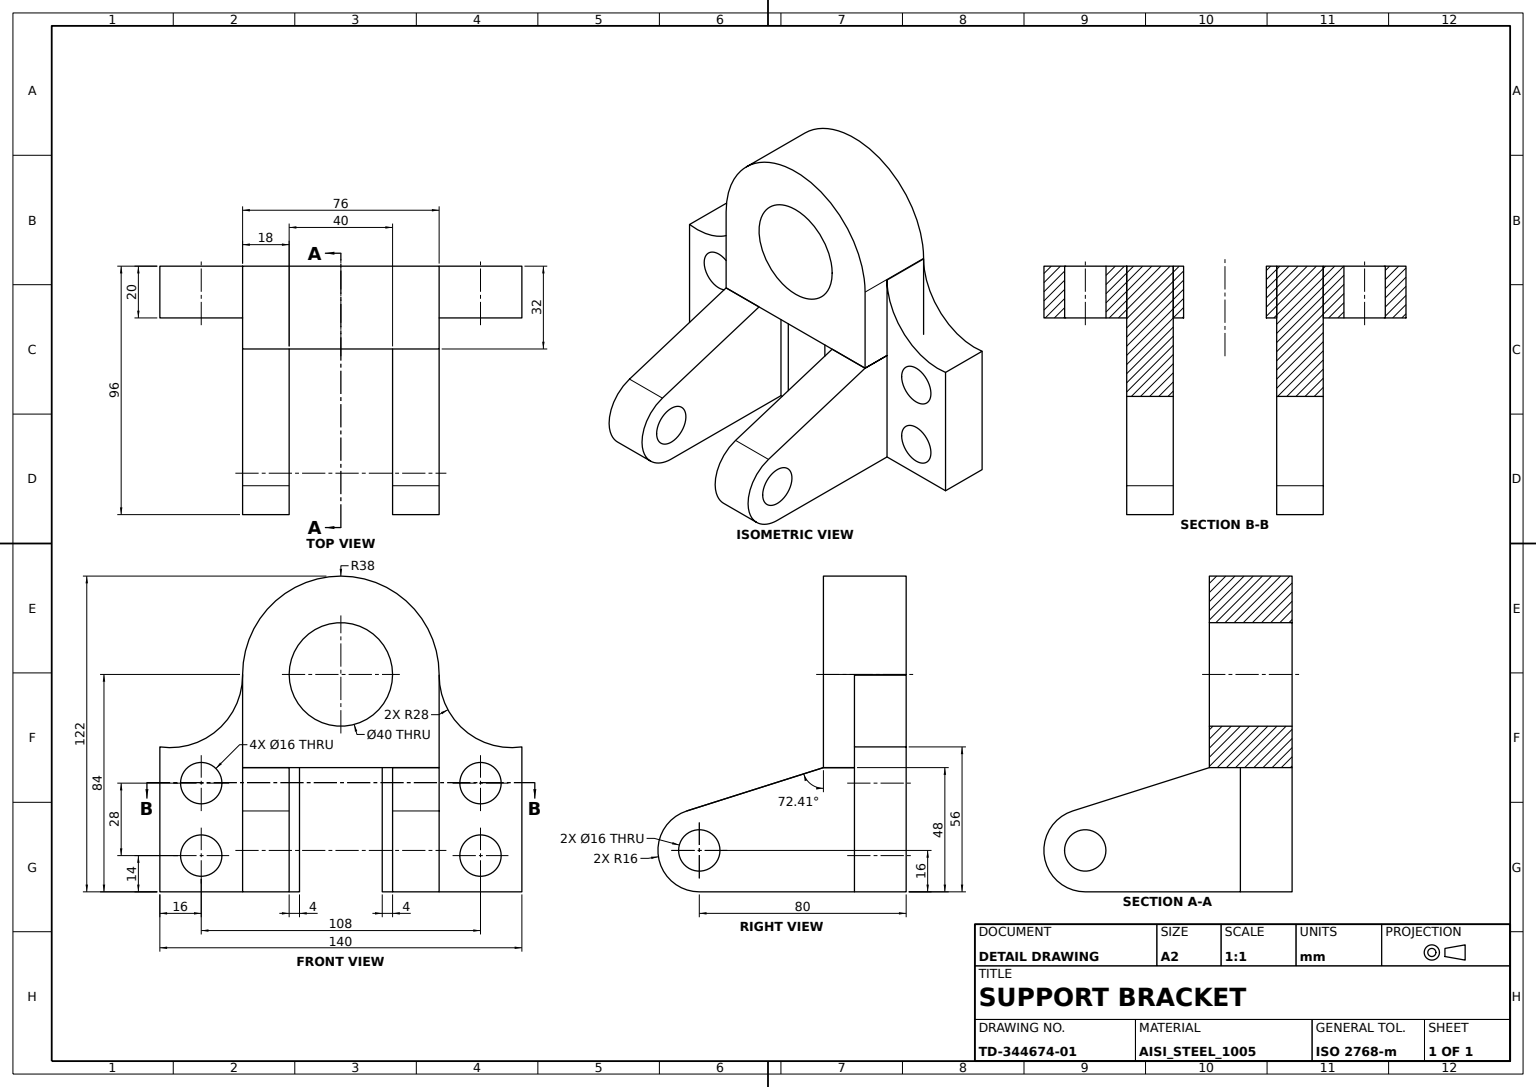
ISO-10303-21;
HEADER;
FILE_DESCRIPTION((''),'2;1');
FILE_NAME('','',(''),(''),'','','');
FILE_SCHEMA(('AUTOMOTIVE_DESIGN'));
ENDSEC;
DATA;
#1=APPLICATION_CONTEXT('');
#2=PRODUCT_CONTEXT('',#1,'mechanical');
#3=PRODUCT('','','',(#2));
#4=PRODUCT_DEFINITION_FORMATION('','',#3);
#5=PRODUCT_DEFINITION_CONTEXT('',#1,'design');
#6=PRODUCT_DEFINITION('','',#4,#5);
#7=PRODUCT_DEFINITION_SHAPE('','',#6);
#8=(LENGTH_UNIT()NAMED_UNIT(*)SI_UNIT(.MILLI.,.METRE.));
#9=(NAMED_UNIT(*)PLANE_ANGLE_UNIT()SI_UNIT($,.RADIAN.));
#10=(NAMED_UNIT(*)SI_UNIT($,.STERADIAN.)SOLID_ANGLE_UNIT());
#11=UNCERTAINTY_MEASURE_WITH_UNIT(LENGTH_MEASURE(0.005),#8,'distance_accuracy_value','');
#12=(GEOMETRIC_REPRESENTATION_CONTEXT(3)GLOBAL_UNCERTAINTY_ASSIGNED_CONTEXT((#11))GLOBAL_UNIT_ASSIGNED_CONTEXT((#8,#9,#10))REPRESENTATION_CONTEXT('',''));
#13=CARTESIAN_POINT('',(20.,-38.,-84.));
#14=VERTEX_POINT('',#13);
#15=CARTESIAN_POINT('',(20.,-70.,-84.));
#16=VERTEX_POINT('',#15);
#17=DIRECTION('',(0.,-1.,0.));
#18=VECTOR('',#17,1000.);
#19=LINE('',#13,#18);
#20=EDGE_CURVE('',#14,#16,#19,.T.);
#21=ORIENTED_EDGE('',*,*,#20,.T.);
#22=CARTESIAN_POINT('',(0.,-70.,-84.));
#23=VERTEX_POINT('',#22);
#24=DIRECTION('',(-1.,0.,0.));
#25=VECTOR('',#24,1000.);
#26=LINE('',#15,#25);
#27=EDGE_CURVE('',#16,#23,#26,.T.);
#28=ORIENTED_EDGE('',*,*,#27,.T.);
#29=CARTESIAN_POINT('',(0.,-38.,-84.));
#30=VERTEX_POINT('',#29);
#31=LINE('',#29,#18);
#32=EDGE_CURVE('',#30,#23,#31,.T.);
#33=ORIENTED_EDGE('',*,*,#32,.F.);
#34=LINE('',#13,#25);
#35=EDGE_CURVE('',#14,#30,#34,.T.);
#36=ORIENTED_EDGE('',*,*,#35,.F.);
#37=EDGE_LOOP('',(#21,#28,#33,#36));
#38=FACE_BOUND('',#37,.T.);
#39=DIRECTION('',(0.,0.,-1.));
#40=AXIS2_PLACEMENT_3D('',#13,#39,#24);
#41=PLANE('',#40);
#42=ADVANCED_FACE('',(#38),#41,.T.);
#43=CARTESIAN_POINT('',(20.,-70.,-28.));
#44=VERTEX_POINT('',#43);
#45=CARTESIAN_POINT('',(0.,-70.,-28.));
#46=VERTEX_POINT('',#45);
#47=LINE('',#43,#25);
#48=EDGE_CURVE('',#44,#46,#47,.T.);
#49=ORIENTED_EDGE('',*,*,#48,.T.);
#50=DIRECTION('',(0.,0.,1.));
#51=VECTOR('',#50,1000.);
#52=LINE('',#22,#51);
#53=EDGE_CURVE('',#23,#46,#52,.T.);
#54=ORIENTED_EDGE('',*,*,#53,.F.);
#55=ORIENTED_EDGE('',*,*,#27,.F.);
#56=LINE('',#15,#51);
#57=EDGE_CURVE('',#16,#44,#56,.T.);
#58=ORIENTED_EDGE('',*,*,#57,.T.);
#59=EDGE_LOOP('',(#49,#54,#55,#58));
#60=FACE_BOUND('',#59,.T.);
#61=AXIS2_PLACEMENT_3D('',#15,#17,#39);
#62=PLANE('',#61);
#63=ADVANCED_FACE('',(#60),#62,.T.);
#64=CARTESIAN_POINT('',(20.,-38.,-0.287187));
#65=VERTEX_POINT('',#64);
#66=CARTESIAN_POINT('',(0.,-38.,-0.287187));
#67=VERTEX_POINT('',#66);
#68=LINE('',#64,#25);
#69=EDGE_CURVE('',#65,#67,#68,.T.);
#70=ORIENTED_EDGE('',*,*,#69,.T.);
#71=CARTESIAN_POINT('',(0.,-66.,-0.287187));
#72=DIRECTION('',(1.,0.,0.));
#73=AXIS2_PLACEMENT_3D('',#71,#72,#17);
#74=CIRCLE('',#73,28.);
#75=EDGE_CURVE('',#46,#67,#74,.T.);
#76=ORIENTED_EDGE('',*,*,#75,.F.);
#77=ORIENTED_EDGE('',*,*,#48,.F.);
#78=CARTESIAN_POINT('',(20.,-66.,-0.287187));
#79=AXIS2_PLACEMENT_3D('',#78,#72,#17);
#80=CIRCLE('',#79,28.);
#81=EDGE_CURVE('',#44,#65,#80,.T.);
#82=ORIENTED_EDGE('',*,*,#81,.T.);
#83=EDGE_LOOP('',(#70,#76,#77,#82));
#84=FACE_BOUND('',#83,.T.);
#85=AXIS2_PLACEMENT_3D('',#78,#24,#50);
#86=CYLINDRICAL_SURFACE('',#85,28.);
#87=ADVANCED_FACE('',(#84),#86,.F.);
#88=ORIENTED_EDGE('',*,*,#69,.F.);
#89=VECTOR('',#39,1000.);
#90=LINE('',#64,#89);
#91=EDGE_CURVE('',#65,#14,#90,.T.);
#92=ORIENTED_EDGE('',*,*,#91,.T.);
#93=ORIENTED_EDGE('',*,*,#35,.T.);
#94=CARTESIAN_POINT('',(0.,-38.,-36.));
#95=LINE('',#94,#89);
#96=EDGE_CURVE('',#67,#30,#95,.T.);
#97=ORIENTED_EDGE('',*,*,#96,.F.);
#98=EDGE_LOOP('',(#88,#92,#93,#97));
#99=FACE_BOUND('',#98,.T.);
#100=CARTESIAN_POINT('',(20.,-38.,-36.));
#101=DIRECTION('',(0.,1.,0.));
#102=AXIS2_PLACEMENT_3D('',#100,#101,#50);
#103=PLANE('',#102);
#104=ADVANCED_FACE('',(#99),#103,.T.);
#105=CARTESIAN_POINT('',(0.,-46.,-42.));
#106=VERTEX_POINT('',#105);
#107=CARTESIAN_POINT('',(0.,-54.,-42.));
#108=AXIS2_PLACEMENT_3D('',#107,#24,#101);
#109=CIRCLE('',#108,8.);
#110=EDGE_CURVE('',#106,#106,#109,.T.);
#111=ORIENTED_EDGE('',*,*,#110,.T.);
#112=EDGE_LOOP('',(#111));
#113=FACE_BOUND('',#112,.T.);
#114=CARTESIAN_POINT('',(20.,-46.,-42.));
#115=VERTEX_POINT('',#114);
#116=CARTESIAN_POINT('',(20.,-54.,-42.));
#117=AXIS2_PLACEMENT_3D('',#116,#24,#101);
#118=CIRCLE('',#117,8.);
#119=EDGE_CURVE('',#115,#115,#118,.T.);
#120=ORIENTED_EDGE('',*,*,#119,.F.);
#121=EDGE_LOOP('',(#120));
#122=FACE_BOUND('',#121,.T.);
#123=AXIS2_PLACEMENT_3D('',#107,#72,#39);
#124=CYLINDRICAL_SURFACE('',#123,8.);
#125=ADVANCED_FACE('',(#113,#122),#124,.F.);
#126=CARTESIAN_POINT('',(20.,-46.,-70.));
#127=VERTEX_POINT('',#126);
#128=CARTESIAN_POINT('',(20.,-54.,-70.));
#129=AXIS2_PLACEMENT_3D('',#128,#24,#101);
#130=CIRCLE('',#129,8.);
#131=EDGE_CURVE('',#127,#127,#130,.T.);
#132=ORIENTED_EDGE('',*,*,#131,.T.);
#133=EDGE_LOOP('',(#132));
#134=FACE_BOUND('',#133,.T.);
#135=ORIENTED_EDGE('',*,*,#119,.T.);
#136=EDGE_LOOP('',(#135));
#137=FACE_BOUND('',#136,.T.);
#138=ORIENTED_EDGE('',*,*,#57,.F.);
#139=ORIENTED_EDGE('',*,*,#20,.F.);
#140=ORIENTED_EDGE('',*,*,#91,.F.);
#141=ORIENTED_EDGE('',*,*,#81,.F.);
#142=EDGE_LOOP('',(#138,#139,#140,#141));
#143=FACE_BOUND('',#142,.T.);
#144=AXIS2_PLACEMENT_3D('',#78,#72,#39);
#145=PLANE('',#144);
#146=ADVANCED_FACE('',(#134,#137,#143),#145,.T.);
#147=ORIENTED_EDGE('',*,*,#131,.F.);
#148=EDGE_LOOP('',(#147));
#149=FACE_BOUND('',#148,.T.);
#150=CARTESIAN_POINT('',(0.,-46.,-70.));
#151=VERTEX_POINT('',#150);
#152=CARTESIAN_POINT('',(0.,-54.,-70.));
#153=AXIS2_PLACEMENT_3D('',#152,#24,#101);
#154=CIRCLE('',#153,8.);
#155=EDGE_CURVE('',#151,#151,#154,.T.);
#156=ORIENTED_EDGE('',*,*,#155,.T.);
#157=EDGE_LOOP('',(#156));
#158=FACE_BOUND('',#157,.T.);
#159=AXIS2_PLACEMENT_3D('',#152,#72,#39);
#160=CYLINDRICAL_SURFACE('',#159,8.);
#161=ADVANCED_FACE('',(#149,#158),#160,.F.);
#162=ORIENTED_EDGE('',*,*,#75,.T.);
#163=ORIENTED_EDGE('',*,*,#96,.T.);
#164=ORIENTED_EDGE('',*,*,#32,.T.);
#165=ORIENTED_EDGE('',*,*,#53,.T.);
#166=EDGE_LOOP('',(#162,#163,#164,#165));
#167=FACE_BOUND('',#166,.T.);
#168=ORIENTED_EDGE('',*,*,#155,.F.);
#169=EDGE_LOOP('',(#168));
#170=FACE_BOUND('',#169,.T.);
#171=ORIENTED_EDGE('',*,*,#110,.F.);
#172=EDGE_LOOP('',(#171));
#173=FACE_BOUND('',#172,.T.);
#174=AXIS2_PLACEMENT_3D('',#71,#72,#39);
#175=PLANE('',#174);
#176=ADVANCED_FACE('',(#167,#170,#173),#175,.F.);
#177=CLOSED_SHELL('',(#42,#63,#87,#104,#125,#146,#161,#176));
#178=MANIFOLD_SOLID_BREP('',#177);
#179=CARTESIAN_POINT('',(0.,-20.,-84.));
#180=VERTEX_POINT('',#179);
#181=CARTESIAN_POINT('',(0.,-20.,-36.));
#182=VERTEX_POINT('',#181);
#183=LINE('',#179,#51);
#184=EDGE_CURVE('',#180,#182,#183,.T.);
#185=ORIENTED_EDGE('',*,*,#184,.F.);
#186=VERTEX_POINT('',#29);
#187=LINE('',#179,#18);
#188=EDGE_CURVE('',#180,#186,#187,.T.);
#189=ORIENTED_EDGE('',*,*,#188,.T.);
#190=VERTEX_POINT('',#94);
#191=LINE('',#29,#51);
#192=EDGE_CURVE('',#186,#190,#191,.T.);
#193=ORIENTED_EDGE('',*,*,#192,.T.);
#194=LINE('',#181,#18);
#195=EDGE_CURVE('',#182,#190,#194,.T.);
#196=ORIENTED_EDGE('',*,*,#195,.F.);
#197=EDGE_LOOP('',(#185,#189,#193,#196));
#198=FACE_BOUND('',#197,.T.);
#199=AXIS2_PLACEMENT_3D('',#179,#72,#39);
#200=PLANE('',#199);
#201=ADVANCED_FACE('',(#198),#200,.F.);
#202=CARTESIAN_POINT('',(84.834712,-20.,-52.747932));
#203=VERTEX_POINT('',#202);
#204=CARTESIAN_POINT('',(84.834712,-38.,-52.747932));
#205=VERTEX_POINT('',#204);
#206=LINE('',#202,#18);
#207=EDGE_CURVE('',#203,#205,#206,.T.);
#208=ORIENTED_EDGE('',*,*,#207,.T.);
#209=CARTESIAN_POINT('',(80.,-38.,-84.));
#210=VERTEX_POINT('',#209);
#211=CARTESIAN_POINT('',(80.,-38.,-68.));
#212=AXIS2_PLACEMENT_3D('',#211,#101,#72);
#213=CIRCLE('',#212,16.);
#214=EDGE_CURVE('',#205,#210,#213,.T.);
#215=ORIENTED_EDGE('',*,*,#214,.T.);
#216=CARTESIAN_POINT('',(80.,-20.,-84.));
#217=VERTEX_POINT('',#216);
#218=LINE('',#216,#18);
#219=EDGE_CURVE('',#217,#210,#218,.T.);
#220=ORIENTED_EDGE('',*,*,#219,.F.);
#221=CARTESIAN_POINT('',(80.,-20.,-68.));
#222=AXIS2_PLACEMENT_3D('',#221,#101,#72);
#223=CIRCLE('',#222,16.);
#224=EDGE_CURVE('',#203,#217,#223,.T.);
#225=ORIENTED_EDGE('',*,*,#224,.F.);
#226=EDGE_LOOP('',(#208,#215,#220,#225));
#227=FACE_BOUND('',#226,.T.);
#228=AXIS2_PLACEMENT_3D('',#221,#17,#39);
#229=CYLINDRICAL_SURFACE('',#228,16.);
#230=ADVANCED_FACE('',(#227),#229,.T.);
#231=CARTESIAN_POINT('',(88.,-20.,-68.));
#232=VERTEX_POINT('',#231);
#233=CIRCLE('',#222,8.);
#234=EDGE_CURVE('',#232,#232,#233,.T.);
#235=ORIENTED_EDGE('',*,*,#234,.F.);
#236=EDGE_LOOP('',(#235));
#237=FACE_BOUND('',#236,.T.);
#238=ORIENTED_EDGE('',*,*,#184,.T.);
#239=CARTESIAN_POINT('',(32.,-20.,-36.));
#240=VERTEX_POINT('',#239);
#241=VECTOR('',#72,1000.);
#242=LINE('',#181,#241);
#243=EDGE_CURVE('',#182,#240,#242,.T.);
#244=ORIENTED_EDGE('',*,*,#243,.T.);
#245=DIRECTION('',(0.953254219,0.,-0.302169479));
#246=VECTOR('',#245,1000.);
#247=LINE('',#239,#246);
#248=EDGE_CURVE('',#240,#203,#247,.T.);
#249=ORIENTED_EDGE('',*,*,#248,.T.);
#250=ORIENTED_EDGE('',*,*,#224,.T.);
#251=LINE('',#216,#25);
#252=EDGE_CURVE('',#217,#180,#251,.T.);
#253=ORIENTED_EDGE('',*,*,#252,.T.);
#254=EDGE_LOOP('',(#238,#244,#249,#250,#253));
#255=FACE_BOUND('',#254,.T.);
#256=AXIS2_PLACEMENT_3D('',#221,#101,#50);
#257=PLANE('',#256);
#258=ADVANCED_FACE('',(#237,#255),#257,.T.);
#259=ORIENTED_EDGE('',*,*,#243,.F.);
#260=ORIENTED_EDGE('',*,*,#195,.T.);
#261=CARTESIAN_POINT('',(32.,-38.,-36.));
#262=VERTEX_POINT('',#261);
#263=LINE('',#94,#241);
#264=EDGE_CURVE('',#190,#262,#263,.T.);
#265=ORIENTED_EDGE('',*,*,#264,.T.);
#266=LINE('',#239,#18);
#267=EDGE_CURVE('',#240,#262,#266,.T.);
#268=ORIENTED_EDGE('',*,*,#267,.F.);
#269=EDGE_LOOP('',(#259,#260,#265,#268));
#270=FACE_BOUND('',#269,.T.);
#271=AXIS2_PLACEMENT_3D('',#181,#39,#24);
#272=PLANE('',#271);
#273=ADVANCED_FACE('',(#270),#272,.F.);
#274=ORIENTED_EDGE('',*,*,#267,.T.);
#275=LINE('',#261,#246);
#276=EDGE_CURVE('',#262,#205,#275,.T.);
#277=ORIENTED_EDGE('',*,*,#276,.T.);
#278=ORIENTED_EDGE('',*,*,#207,.F.);
#279=ORIENTED_EDGE('',*,*,#248,.F.);
#280=EDGE_LOOP('',(#274,#277,#278,#279));
#281=FACE_BOUND('',#280,.T.);
#282=DIRECTION('',(-0.302169479,0.,-0.953254219));
#283=DIRECTION('',(-0.953254219,0.,0.302169479));
#284=AXIS2_PLACEMENT_3D('',#239,#282,#283);
#285=PLANE('',#284);
#286=ADVANCED_FACE('',(#281),#285,.F.);
#287=CARTESIAN_POINT('',(88.,-38.,-68.));
#288=VERTEX_POINT('',#287);
#289=CIRCLE('',#212,8.);
#290=EDGE_CURVE('',#288,#288,#289,.T.);
#291=ORIENTED_EDGE('',*,*,#290,.F.);
#292=EDGE_LOOP('',(#291));
#293=FACE_BOUND('',#292,.T.);
#294=ORIENTED_EDGE('',*,*,#234,.T.);
#295=EDGE_LOOP('',(#294));
#296=FACE_BOUND('',#295,.T.);
#297=CYLINDRICAL_SURFACE('',#228,8.);
#298=ADVANCED_FACE('',(#293,#296),#297,.F.);
#299=ORIENTED_EDGE('',*,*,#188,.F.);
#300=ORIENTED_EDGE('',*,*,#252,.F.);
#301=ORIENTED_EDGE('',*,*,#219,.T.);
#302=LINE('',#209,#25);
#303=EDGE_CURVE('',#210,#186,#302,.T.);
#304=ORIENTED_EDGE('',*,*,#303,.T.);
#305=EDGE_LOOP('',(#299,#300,#301,#304));
#306=FACE_BOUND('',#305,.T.);
#307=AXIS2_PLACEMENT_3D('',#216,#50,#72);
#308=PLANE('',#307);
#309=ADVANCED_FACE('',(#306),#308,.F.);
#310=ORIENTED_EDGE('',*,*,#303,.F.);
#311=ORIENTED_EDGE('',*,*,#214,.F.);
#312=ORIENTED_EDGE('',*,*,#276,.F.);
#313=ORIENTED_EDGE('',*,*,#264,.F.);
#314=ORIENTED_EDGE('',*,*,#192,.F.);
#315=EDGE_LOOP('',(#310,#311,#312,#313,#314));
#316=FACE_BOUND('',#315,.T.);
#317=ORIENTED_EDGE('',*,*,#290,.T.);
#318=EDGE_LOOP('',(#317));
#319=FACE_BOUND('',#318,.T.);
#320=AXIS2_PLACEMENT_3D('',#211,#101,#50);
#321=PLANE('',#320);
#322=ADVANCED_FACE('',(#316,#319),#321,.F.);
#323=CLOSED_SHELL('',(#201,#230,#258,#273,#286,#298,#309,#322));
#324=MANIFOLD_SOLID_BREP('',#323);
#325=CARTESIAN_POINT('',(84.834712,20.,-52.747932));
#326=VERTEX_POINT('',#325);
#327=CARTESIAN_POINT('',(80.,20.,-84.));
#328=VERTEX_POINT('',#327);
#329=CARTESIAN_POINT('',(80.,20.,-68.));
#330=AXIS2_PLACEMENT_3D('',#329,#101,#72);
#331=CIRCLE('',#330,16.);
#332=EDGE_CURVE('',#326,#328,#331,.T.);
#333=ORIENTED_EDGE('',*,*,#332,.F.);
#334=CARTESIAN_POINT('',(32.,20.,-36.));
#335=VERTEX_POINT('',#334);
#336=LINE('',#334,#246);
#337=EDGE_CURVE('',#335,#326,#336,.T.);
#338=ORIENTED_EDGE('',*,*,#337,.F.);
#339=CARTESIAN_POINT('',(0.,20.,-36.));
#340=VERTEX_POINT('',#339);
#341=LINE('',#339,#241);
#342=EDGE_CURVE('',#340,#335,#341,.T.);
#343=ORIENTED_EDGE('',*,*,#342,.F.);
#344=CARTESIAN_POINT('',(0.,20.,-84.));
#345=VERTEX_POINT('',#344);
#346=LINE('',#344,#51);
#347=EDGE_CURVE('',#345,#340,#346,.T.);
#348=ORIENTED_EDGE('',*,*,#347,.F.);
#349=LINE('',#327,#25);
#350=EDGE_CURVE('',#328,#345,#349,.T.);
#351=ORIENTED_EDGE('',*,*,#350,.F.);
#352=EDGE_LOOP('',(#333,#338,#343,#348,#351));
#353=FACE_BOUND('',#352,.T.);
#354=CARTESIAN_POINT('',(88.,20.,-68.));
#355=VERTEX_POINT('',#354);
#356=CIRCLE('',#330,8.);
#357=EDGE_CURVE('',#355,#355,#356,.T.);
#358=ORIENTED_EDGE('',*,*,#357,.T.);
#359=EDGE_LOOP('',(#358));
#360=FACE_BOUND('',#359,.T.);
#361=AXIS2_PLACEMENT_3D('',#329,#101,#50);
#362=PLANE('',#361);
#363=ADVANCED_FACE('',(#353,#360),#362,.F.);
#364=ORIENTED_EDGE('',*,*,#347,.T.);
#365=CARTESIAN_POINT('',(0.,38.,-36.));
#366=VERTEX_POINT('',#365);
#367=VECTOR('',#101,1000.);
#368=LINE('',#339,#367);
#369=EDGE_CURVE('',#340,#366,#368,.T.);
#370=ORIENTED_EDGE('',*,*,#369,.T.);
#371=CARTESIAN_POINT('',(0.,38.,-84.));
#372=VERTEX_POINT('',#371);
#373=LINE('',#371,#51);
#374=EDGE_CURVE('',#372,#366,#373,.T.);
#375=ORIENTED_EDGE('',*,*,#374,.F.);
#376=LINE('',#344,#367);
#377=EDGE_CURVE('',#345,#372,#376,.T.);
#378=ORIENTED_EDGE('',*,*,#377,.F.);
#379=EDGE_LOOP('',(#364,#370,#375,#378));
#380=FACE_BOUND('',#379,.T.);
#381=AXIS2_PLACEMENT_3D('',#344,#24,#50);
#382=PLANE('',#381);
#383=ADVANCED_FACE('',(#380),#382,.T.);
#384=CARTESIAN_POINT('',(88.,38.,-68.));
#385=VERTEX_POINT('',#384);
#386=CARTESIAN_POINT('',(80.,38.,-68.));
#387=AXIS2_PLACEMENT_3D('',#386,#101,#72);
#388=CIRCLE('',#387,8.);
#389=EDGE_CURVE('',#385,#385,#388,.T.);
#390=ORIENTED_EDGE('',*,*,#389,.T.);
#391=EDGE_LOOP('',(#390));
#392=FACE_BOUND('',#391,.T.);
#393=ORIENTED_EDGE('',*,*,#357,.F.);
#394=EDGE_LOOP('',(#393));
#395=FACE_BOUND('',#394,.T.);
#396=CYLINDRICAL_SURFACE('',#361,8.);
#397=ADVANCED_FACE('',(#392,#395),#396,.F.);
#398=CARTESIAN_POINT('',(80.,38.,-84.));
#399=VERTEX_POINT('',#398);
#400=LINE('',#327,#367);
#401=EDGE_CURVE('',#328,#399,#400,.T.);
#402=ORIENTED_EDGE('',*,*,#401,.T.);
#403=CARTESIAN_POINT('',(84.834712,38.,-52.747932));
#404=VERTEX_POINT('',#403);
#405=CIRCLE('',#387,16.);
#406=EDGE_CURVE('',#404,#399,#405,.T.);
#407=ORIENTED_EDGE('',*,*,#406,.F.);
#408=LINE('',#325,#367);
#409=EDGE_CURVE('',#326,#404,#408,.T.);
#410=ORIENTED_EDGE('',*,*,#409,.F.);
#411=ORIENTED_EDGE('',*,*,#332,.T.);
#412=EDGE_LOOP('',(#402,#407,#410,#411));
#413=FACE_BOUND('',#412,.T.);
#414=CYLINDRICAL_SURFACE('',#361,16.);
#415=ADVANCED_FACE('',(#413),#414,.T.);
#416=ORIENTED_EDGE('',*,*,#369,.F.);
#417=ORIENTED_EDGE('',*,*,#342,.T.);
#418=CARTESIAN_POINT('',(32.,38.,-36.));
#419=VERTEX_POINT('',#418);
#420=LINE('',#334,#367);
#421=EDGE_CURVE('',#335,#419,#420,.T.);
#422=ORIENTED_EDGE('',*,*,#421,.T.);
#423=LINE('',#365,#241);
#424=EDGE_CURVE('',#366,#419,#423,.T.);
#425=ORIENTED_EDGE('',*,*,#424,.F.);
#426=EDGE_LOOP('',(#416,#417,#422,#425));
#427=FACE_BOUND('',#426,.T.);
#428=AXIS2_PLACEMENT_3D('',#339,#50,#72);
#429=PLANE('',#428);
#430=ADVANCED_FACE('',(#427),#429,.T.);
#431=ORIENTED_EDGE('',*,*,#377,.T.);
#432=LINE('',#398,#25);
#433=EDGE_CURVE('',#399,#372,#432,.T.);
#434=ORIENTED_EDGE('',*,*,#433,.F.);
#435=ORIENTED_EDGE('',*,*,#401,.F.);
#436=ORIENTED_EDGE('',*,*,#350,.T.);
#437=EDGE_LOOP('',(#431,#434,#435,#436));
#438=FACE_BOUND('',#437,.T.);
#439=AXIS2_PLACEMENT_3D('',#327,#39,#24);
#440=PLANE('',#439);
#441=ADVANCED_FACE('',(#438),#440,.T.);
#442=ORIENTED_EDGE('',*,*,#409,.T.);
#443=LINE('',#418,#246);
#444=EDGE_CURVE('',#419,#404,#443,.T.);
#445=ORIENTED_EDGE('',*,*,#444,.F.);
#446=ORIENTED_EDGE('',*,*,#421,.F.);
#447=ORIENTED_EDGE('',*,*,#337,.T.);
#448=EDGE_LOOP('',(#442,#445,#446,#447));
#449=FACE_BOUND('',#448,.T.);
#450=DIRECTION('',(0.302169479,0.,0.953254219));
#451=AXIS2_PLACEMENT_3D('',#334,#450,#245);
#452=PLANE('',#451);
#453=ADVANCED_FACE('',(#449),#452,.T.);
#454=ORIENTED_EDGE('',*,*,#389,.F.);
#455=EDGE_LOOP('',(#454));
#456=FACE_BOUND('',#455,.T.);
#457=ORIENTED_EDGE('',*,*,#433,.T.);
#458=ORIENTED_EDGE('',*,*,#374,.T.);
#459=ORIENTED_EDGE('',*,*,#424,.T.);
#460=ORIENTED_EDGE('',*,*,#444,.T.);
#461=ORIENTED_EDGE('',*,*,#406,.T.);
#462=EDGE_LOOP('',(#457,#458,#459,#460,#461));
#463=FACE_BOUND('',#462,.T.);
#464=AXIS2_PLACEMENT_3D('',#386,#101,#50);
#465=PLANE('',#464);
#466=ADVANCED_FACE('',(#456,#463),#465,.T.);
#467=CLOSED_SHELL('',(#363,#383,#397,#415,#430,#441,#453,#466));
#468=MANIFOLD_SOLID_BREP('',#467);
#469=CARTESIAN_POINT('',(0.,-38.,0.));
#470=VERTEX_POINT('',#469);
#471=CARTESIAN_POINT('',(0.,38.,0.));
#472=VERTEX_POINT('',#471);
#473=CARTESIAN_POINT('',(0.,0.,0.));
#474=AXIS2_PLACEMENT_3D('',#473,#24,#101);
#475=CIRCLE('',#474,38.);
#476=EDGE_CURVE('',#470,#472,#475,.T.);
#477=ORIENTED_EDGE('',*,*,#476,.F.);
#478=CARTESIAN_POINT('',(32.,-38.,0.));
#479=VERTEX_POINT('',#478);
#480=LINE('',#478,#25);
#481=EDGE_CURVE('',#479,#470,#480,.T.);
#482=ORIENTED_EDGE('',*,*,#481,.F.);
#483=CARTESIAN_POINT('',(32.,38.,0.));
#484=VERTEX_POINT('',#483);
#485=CARTESIAN_POINT('',(32.,0.,0.));
#486=AXIS2_PLACEMENT_3D('',#485,#24,#101);
#487=CIRCLE('',#486,38.);
#488=EDGE_CURVE('',#479,#484,#487,.T.);
#489=ORIENTED_EDGE('',*,*,#488,.T.);
#490=LINE('',#483,#25);
#491=EDGE_CURVE('',#484,#472,#490,.T.);
#492=ORIENTED_EDGE('',*,*,#491,.T.);
#493=EDGE_LOOP('',(#477,#482,#489,#492));
#494=FACE_BOUND('',#493,.T.);
#495=AXIS2_PLACEMENT_3D('',#485,#24,#50);
#496=CYLINDRICAL_SURFACE('',#495,38.);
#497=ADVANCED_FACE('',(#494),#496,.T.);
#498=CARTESIAN_POINT('',(32.,20.,0.));
#499=VERTEX_POINT('',#498);
#500=CIRCLE('',#486,20.);
#501=EDGE_CURVE('',#499,#499,#500,.T.);
#502=ORIENTED_EDGE('',*,*,#501,.T.);
#503=EDGE_LOOP('',(#502));
#504=FACE_BOUND('',#503,.T.);
#505=ORIENTED_EDGE('',*,*,#488,.F.);
#506=VERTEX_POINT('',#261);
#507=LINE('',#261,#51);
#508=EDGE_CURVE('',#506,#479,#507,.T.);
#509=ORIENTED_EDGE('',*,*,#508,.F.);
#510=VERTEX_POINT('',#418);
#511=LINE('',#418,#18);
#512=EDGE_CURVE('',#510,#506,#511,.T.);
#513=ORIENTED_EDGE('',*,*,#512,.F.);
#514=LINE('',#483,#89);
#515=EDGE_CURVE('',#484,#510,#514,.T.);
#516=ORIENTED_EDGE('',*,*,#515,.F.);
#517=EDGE_LOOP('',(#505,#509,#513,#516));
#518=FACE_BOUND('',#517,.T.);
#519=PLANE('',#495);
#520=ADVANCED_FACE('',(#504,#518),#519,.F.);
#521=VERTEX_POINT('',#365);
#522=LINE('',#471,#89);
#523=EDGE_CURVE('',#472,#521,#522,.T.);
#524=ORIENTED_EDGE('',*,*,#523,.F.);
#525=ORIENTED_EDGE('',*,*,#491,.F.);
#526=ORIENTED_EDGE('',*,*,#515,.T.);
#527=LINE('',#418,#25);
#528=EDGE_CURVE('',#510,#521,#527,.T.);
#529=ORIENTED_EDGE('',*,*,#528,.T.);
#530=EDGE_LOOP('',(#524,#525,#526,#529));
#531=FACE_BOUND('',#530,.T.);
#532=AXIS2_PLACEMENT_3D('',#483,#101,#50);
#533=PLANE('',#532);
#534=ADVANCED_FACE('',(#531),#533,.T.);
#535=VERTEX_POINT('',#94);
#536=LINE('',#261,#25);
#537=EDGE_CURVE('',#506,#535,#536,.T.);
#538=ORIENTED_EDGE('',*,*,#537,.T.);
#539=LINE('',#365,#18);
#540=EDGE_CURVE('',#521,#535,#539,.T.);
#541=ORIENTED_EDGE('',*,*,#540,.F.);
#542=ORIENTED_EDGE('',*,*,#528,.F.);
#543=ORIENTED_EDGE('',*,*,#512,.T.);
#544=EDGE_LOOP('',(#538,#541,#542,#543));
#545=FACE_BOUND('',#544,.T.);
#546=AXIS2_PLACEMENT_3D('',#418,#39,#24);
#547=PLANE('',#546);
#548=ADVANCED_FACE('',(#545),#547,.T.);
#549=ORIENTED_EDGE('',*,*,#481,.T.);
#550=LINE('',#94,#51);
#551=EDGE_CURVE('',#535,#470,#550,.T.);
#552=ORIENTED_EDGE('',*,*,#551,.F.);
#553=ORIENTED_EDGE('',*,*,#537,.F.);
#554=ORIENTED_EDGE('',*,*,#508,.T.);
#555=EDGE_LOOP('',(#549,#552,#553,#554));
#556=FACE_BOUND('',#555,.T.);
#557=AXIS2_PLACEMENT_3D('',#261,#17,#39);
#558=PLANE('',#557);
#559=ADVANCED_FACE('',(#556),#558,.T.);
#560=ORIENTED_EDGE('',*,*,#501,.F.);
#561=EDGE_LOOP('',(#560));
#562=FACE_BOUND('',#561,.T.);
#563=CARTESIAN_POINT('',(0.,20.,0.));
#564=VERTEX_POINT('',#563);
#565=CIRCLE('',#474,20.);
#566=EDGE_CURVE('',#564,#564,#565,.T.);
#567=ORIENTED_EDGE('',*,*,#566,.T.);
#568=EDGE_LOOP('',(#567));
#569=FACE_BOUND('',#568,.T.);
#570=CYLINDRICAL_SURFACE('',#495,20.);
#571=ADVANCED_FACE('',(#562,#569),#570,.F.);
#572=ORIENTED_EDGE('',*,*,#523,.T.);
#573=ORIENTED_EDGE('',*,*,#540,.T.);
#574=ORIENTED_EDGE('',*,*,#551,.T.);
#575=ORIENTED_EDGE('',*,*,#476,.T.);
#576=EDGE_LOOP('',(#572,#573,#574,#575));
#577=FACE_BOUND('',#576,.T.);
#578=ORIENTED_EDGE('',*,*,#566,.F.);
#579=EDGE_LOOP('',(#578));
#580=FACE_BOUND('',#579,.T.);
#581=AXIS2_PLACEMENT_3D('',#473,#24,#50);
#582=PLANE('',#581);
#583=ADVANCED_FACE('',(#577,#580),#582,.T.);
#584=CLOSED_SHELL('',(#497,#520,#534,#548,#559,#571,#583));
#585=MANIFOLD_SOLID_BREP('',#584);
#586=CARTESIAN_POINT('',(0.,-16.,-84.));
#587=VERTEX_POINT('',#586);
#588=CARTESIAN_POINT('',(20.,-16.,-84.));
#589=VERTEX_POINT('',#588);
#590=LINE('',#586,#241);
#591=EDGE_CURVE('',#587,#589,#590,.T.);
#592=ORIENTED_EDGE('',*,*,#591,.F.);
#593=CARTESIAN_POINT('',(0.,-16.,-36.));
#594=VERTEX_POINT('',#593);
#595=LINE('',#593,#89);
#596=EDGE_CURVE('',#594,#587,#595,.T.);
#597=ORIENTED_EDGE('',*,*,#596,.F.);
#598=CARTESIAN_POINT('',(20.,-16.,-36.));
#599=VERTEX_POINT('',#598);
#600=LINE('',#598,#25);
#601=EDGE_CURVE('',#599,#594,#600,.T.);
#602=ORIENTED_EDGE('',*,*,#601,.F.);
#603=LINE('',#588,#51);
#604=EDGE_CURVE('',#589,#599,#603,.T.);
#605=ORIENTED_EDGE('',*,*,#604,.F.);
#606=EDGE_LOOP('',(#592,#597,#602,#605));
#607=FACE_BOUND('',#606,.T.);
#608=CARTESIAN_POINT('',(0.,-16.,0.));
#609=AXIS2_PLACEMENT_3D('',#608,#17,#39);
#610=PLANE('',#609);
#611=ADVANCED_FACE('',(#607),#610,.F.);
#612=CARTESIAN_POINT('',(20.,-20.,-36.));
#613=VERTEX_POINT('',#612);
#614=LINE('',#598,#18);
#615=EDGE_CURVE('',#599,#613,#614,.T.);
#616=ORIENTED_EDGE('',*,*,#615,.F.);
#617=ORIENTED_EDGE('',*,*,#601,.T.);
#618=VERTEX_POINT('',#181);
#619=LINE('',#593,#18);
#620=EDGE_CURVE('',#594,#618,#619,.T.);
#621=ORIENTED_EDGE('',*,*,#620,.T.);
#622=LINE('',#612,#25);
#623=EDGE_CURVE('',#613,#618,#622,.T.);
#624=ORIENTED_EDGE('',*,*,#623,.F.);
#625=EDGE_LOOP('',(#616,#617,#621,#624));
#626=FACE_BOUND('',#625,.T.);
#627=AXIS2_PLACEMENT_3D('',#598,#50,#72);
#628=PLANE('',#627);
#629=ADVANCED_FACE('',(#626),#628,.T.);
#630=ORIENTED_EDGE('',*,*,#620,.F.);
#631=ORIENTED_EDGE('',*,*,#596,.T.);
#632=VERTEX_POINT('',#179);
#633=LINE('',#586,#18);
#634=EDGE_CURVE('',#587,#632,#633,.T.);
#635=ORIENTED_EDGE('',*,*,#634,.T.);
#636=LINE('',#181,#89);
#637=EDGE_CURVE('',#618,#632,#636,.T.);
#638=ORIENTED_EDGE('',*,*,#637,.F.);
#639=EDGE_LOOP('',(#630,#631,#635,#638));
#640=FACE_BOUND('',#639,.T.);
#641=AXIS2_PLACEMENT_3D('',#593,#24,#50);
#642=PLANE('',#641);
#643=ADVANCED_FACE('',(#640),#642,.T.);
#644=CARTESIAN_POINT('',(20.,-20.,-84.));
#645=VERTEX_POINT('',#644);
#646=LINE('',#644,#51);
#647=EDGE_CURVE('',#645,#613,#646,.T.);
#648=ORIENTED_EDGE('',*,*,#647,.F.);
#649=LINE('',#588,#18);
#650=EDGE_CURVE('',#589,#645,#649,.T.);
#651=ORIENTED_EDGE('',*,*,#650,.F.);
#652=ORIENTED_EDGE('',*,*,#604,.T.);
#653=ORIENTED_EDGE('',*,*,#615,.T.);
#654=EDGE_LOOP('',(#648,#651,#652,#653));
#655=FACE_BOUND('',#654,.T.);
#656=AXIS2_PLACEMENT_3D('',#588,#72,#39);
#657=PLANE('',#656);
#658=ADVANCED_FACE('',(#655),#657,.T.);
#659=ORIENTED_EDGE('',*,*,#623,.T.);
#660=ORIENTED_EDGE('',*,*,#637,.T.);
#661=LINE('',#179,#241);
#662=EDGE_CURVE('',#632,#645,#661,.T.);
#663=ORIENTED_EDGE('',*,*,#662,.T.);
#664=ORIENTED_EDGE('',*,*,#647,.T.);
#665=EDGE_LOOP('',(#659,#660,#663,#664));
#666=FACE_BOUND('',#665,.T.);
#667=CARTESIAN_POINT('',(0.,-20.,0.));
#668=AXIS2_PLACEMENT_3D('',#667,#17,#39);
#669=PLANE('',#668);
#670=ADVANCED_FACE('',(#666),#669,.T.);
#671=ORIENTED_EDGE('',*,*,#650,.T.);
#672=ORIENTED_EDGE('',*,*,#662,.F.);
#673=ORIENTED_EDGE('',*,*,#634,.F.);
#674=ORIENTED_EDGE('',*,*,#591,.T.);
#675=EDGE_LOOP('',(#671,#672,#673,#674));
#676=FACE_BOUND('',#675,.T.);
#677=AXIS2_PLACEMENT_3D('',#586,#39,#24);
#678=PLANE('',#677);
#679=ADVANCED_FACE('',(#676),#678,.T.);
#680=CLOSED_SHELL('',(#611,#629,#643,#658,#670,#679));
#681=MANIFOLD_SOLID_BREP('',#680);
#682=CARTESIAN_POINT('',(0.,16.,-84.));
#683=VERTEX_POINT('',#682);
#684=CARTESIAN_POINT('',(20.,16.,-84.));
#685=VERTEX_POINT('',#684);
#686=LINE('',#682,#241);
#687=EDGE_CURVE('',#683,#685,#686,.T.);
#688=ORIENTED_EDGE('',*,*,#687,.F.);
#689=VERTEX_POINT('',#344);
#690=LINE('',#682,#367);
#691=EDGE_CURVE('',#683,#689,#690,.T.);
#692=ORIENTED_EDGE('',*,*,#691,.T.);
#693=CARTESIAN_POINT('',(20.,20.,-84.));
#694=VERTEX_POINT('',#693);
#695=LINE('',#344,#241);
#696=EDGE_CURVE('',#689,#694,#695,.T.);
#697=ORIENTED_EDGE('',*,*,#696,.T.);
#698=LINE('',#684,#367);
#699=EDGE_CURVE('',#685,#694,#698,.T.);
#700=ORIENTED_EDGE('',*,*,#699,.F.);
#701=EDGE_LOOP('',(#688,#692,#697,#700));
#702=FACE_BOUND('',#701,.T.);
#703=AXIS2_PLACEMENT_3D('',#682,#50,#72);
#704=PLANE('',#703);
#705=ADVANCED_FACE('',(#702),#704,.F.);
#706=CARTESIAN_POINT('',(20.,16.,-36.));
#707=VERTEX_POINT('',#706);
#708=CARTESIAN_POINT('',(0.,16.,-36.));
#709=VERTEX_POINT('',#708);
#710=LINE('',#706,#25);
#711=EDGE_CURVE('',#707,#709,#710,.T.);
#712=ORIENTED_EDGE('',*,*,#711,.T.);
#713=LINE('',#708,#89);
#714=EDGE_CURVE('',#709,#683,#713,.T.);
#715=ORIENTED_EDGE('',*,*,#714,.T.);
#716=ORIENTED_EDGE('',*,*,#687,.T.);
#717=LINE('',#684,#51);
#718=EDGE_CURVE('',#685,#707,#717,.T.);
#719=ORIENTED_EDGE('',*,*,#718,.T.);
#720=EDGE_LOOP('',(#712,#715,#716,#719));
#721=FACE_BOUND('',#720,.T.);
#722=CARTESIAN_POINT('',(0.,16.,0.));
#723=AXIS2_PLACEMENT_3D('',#722,#17,#39);
#724=PLANE('',#723);
#725=ADVANCED_FACE('',(#721),#724,.T.);
#726=CARTESIAN_POINT('',(20.,20.,-36.));
#727=VERTEX_POINT('',#726);
#728=LINE('',#693,#51);
#729=EDGE_CURVE('',#694,#727,#728,.T.);
#730=ORIENTED_EDGE('',*,*,#729,.T.);
#731=LINE('',#706,#367);
#732=EDGE_CURVE('',#707,#727,#731,.T.);
#733=ORIENTED_EDGE('',*,*,#732,.F.);
#734=ORIENTED_EDGE('',*,*,#718,.F.);
#735=ORIENTED_EDGE('',*,*,#699,.T.);
#736=EDGE_LOOP('',(#730,#733,#734,#735));
#737=FACE_BOUND('',#736,.T.);
#738=AXIS2_PLACEMENT_3D('',#684,#24,#50);
#739=PLANE('',#738);
#740=ADVANCED_FACE('',(#737),#739,.F.);
#741=ORIENTED_EDGE('',*,*,#729,.F.);
#742=ORIENTED_EDGE('',*,*,#696,.F.);
#743=VERTEX_POINT('',#339);
#744=LINE('',#339,#89);
#745=EDGE_CURVE('',#743,#689,#744,.T.);
#746=ORIENTED_EDGE('',*,*,#745,.F.);
#747=LINE('',#726,#25);
#748=EDGE_CURVE('',#727,#743,#747,.T.);
#749=ORIENTED_EDGE('',*,*,#748,.F.);
#750=EDGE_LOOP('',(#741,#742,#746,#749));
#751=FACE_BOUND('',#750,.T.);
#752=AXIS2_PLACEMENT_3D('',#563,#17,#39);
#753=PLANE('',#752);
#754=ADVANCED_FACE('',(#751),#753,.F.);
#755=ORIENTED_EDGE('',*,*,#745,.T.);
#756=ORIENTED_EDGE('',*,*,#691,.F.);
#757=ORIENTED_EDGE('',*,*,#714,.F.);
#758=LINE('',#708,#367);
#759=EDGE_CURVE('',#709,#743,#758,.T.);
#760=ORIENTED_EDGE('',*,*,#759,.T.);
#761=EDGE_LOOP('',(#755,#756,#757,#760));
#762=FACE_BOUND('',#761,.T.);
#763=AXIS2_PLACEMENT_3D('',#708,#72,#39);
#764=PLANE('',#763);
#765=ADVANCED_FACE('',(#762),#764,.F.);
#766=ORIENTED_EDGE('',*,*,#732,.T.);
#767=ORIENTED_EDGE('',*,*,#748,.T.);
#768=ORIENTED_EDGE('',*,*,#759,.F.);
#769=ORIENTED_EDGE('',*,*,#711,.F.);
#770=EDGE_LOOP('',(#766,#767,#768,#769));
#771=FACE_BOUND('',#770,.T.);
#772=AXIS2_PLACEMENT_3D('',#706,#39,#24);
#773=PLANE('',#772);
#774=ADVANCED_FACE('',(#771),#773,.F.);
#775=CLOSED_SHELL('',(#705,#725,#740,#754,#765,#774));
#776=MANIFOLD_SOLID_BREP('',#775);
#777=CARTESIAN_POINT('',(20.,38.,-0.287187));
#778=VERTEX_POINT('',#777);
#779=CARTESIAN_POINT('',(20.,38.,-84.));
#780=VERTEX_POINT('',#779);
#781=LINE('',#777,#89);
#782=EDGE_CURVE('',#778,#780,#781,.T.);
#783=ORIENTED_EDGE('',*,*,#782,.T.);
#784=CARTESIAN_POINT('',(20.,70.,-84.));
#785=VERTEX_POINT('',#784);
#786=LINE('',#779,#367);
#787=EDGE_CURVE('',#780,#785,#786,.T.);
#788=ORIENTED_EDGE('',*,*,#787,.T.);
#789=CARTESIAN_POINT('',(20.,70.,-28.));
#790=VERTEX_POINT('',#789);
#791=LINE('',#784,#51);
#792=EDGE_CURVE('',#785,#790,#791,.T.);
#793=ORIENTED_EDGE('',*,*,#792,.T.);
#794=CARTESIAN_POINT('',(20.,66.,-0.287187));
#795=AXIS2_PLACEMENT_3D('',#794,#24,#101);
#796=CIRCLE('',#795,28.);
#797=EDGE_CURVE('',#790,#778,#796,.T.);
#798=ORIENTED_EDGE('',*,*,#797,.T.);
#799=EDGE_LOOP('',(#783,#788,#793,#798));
#800=FACE_BOUND('',#799,.T.);
#801=CARTESIAN_POINT('',(20.,46.,-70.));
#802=VERTEX_POINT('',#801);
#803=CARTESIAN_POINT('',(20.,54.,-70.));
#804=AXIS2_PLACEMENT_3D('',#803,#72,#17);
#805=CIRCLE('',#804,8.);
#806=EDGE_CURVE('',#802,#802,#805,.T.);
#807=ORIENTED_EDGE('',*,*,#806,.F.);
#808=EDGE_LOOP('',(#807));
#809=FACE_BOUND('',#808,.T.);
#810=CARTESIAN_POINT('',(20.,46.,-42.));
#811=VERTEX_POINT('',#810);
#812=CARTESIAN_POINT('',(20.,54.,-42.));
#813=AXIS2_PLACEMENT_3D('',#812,#72,#17);
#814=CIRCLE('',#813,8.);
#815=EDGE_CURVE('',#811,#811,#814,.T.);
#816=ORIENTED_EDGE('',*,*,#815,.F.);
#817=EDGE_LOOP('',(#816));
#818=FACE_BOUND('',#817,.T.);
#819=AXIS2_PLACEMENT_3D('',#794,#24,#50);
#820=PLANE('',#819);
#821=ADVANCED_FACE('',(#800,#809,#818),#820,.F.);
#822=CARTESIAN_POINT('',(0.,70.,-28.));
#823=VERTEX_POINT('',#822);
#824=CARTESIAN_POINT('',(0.,38.,-0.287187));
#825=VERTEX_POINT('',#824);
#826=CARTESIAN_POINT('',(0.,66.,-0.287187));
#827=AXIS2_PLACEMENT_3D('',#826,#24,#101);
#828=CIRCLE('',#827,28.);
#829=EDGE_CURVE('',#823,#825,#828,.T.);
#830=ORIENTED_EDGE('',*,*,#829,.F.);
#831=CARTESIAN_POINT('',(0.,70.,-84.));
#832=VERTEX_POINT('',#831);
#833=LINE('',#831,#51);
#834=EDGE_CURVE('',#832,#823,#833,.T.);
#835=ORIENTED_EDGE('',*,*,#834,.F.);
#836=VERTEX_POINT('',#371);
#837=LINE('',#371,#367);
#838=EDGE_CURVE('',#836,#832,#837,.T.);
#839=ORIENTED_EDGE('',*,*,#838,.F.);
#840=LINE('',#365,#89);
#841=EDGE_CURVE('',#825,#836,#840,.T.);
#842=ORIENTED_EDGE('',*,*,#841,.F.);
#843=EDGE_LOOP('',(#830,#835,#839,#842));
#844=FACE_BOUND('',#843,.T.);
#845=CARTESIAN_POINT('',(0.,46.,-42.));
#846=VERTEX_POINT('',#845);
#847=CARTESIAN_POINT('',(0.,54.,-42.));
#848=AXIS2_PLACEMENT_3D('',#847,#72,#17);
#849=CIRCLE('',#848,8.);
#850=EDGE_CURVE('',#846,#846,#849,.T.);
#851=ORIENTED_EDGE('',*,*,#850,.T.);
#852=EDGE_LOOP('',(#851));
#853=FACE_BOUND('',#852,.T.);
#854=CARTESIAN_POINT('',(0.,46.,-70.));
#855=VERTEX_POINT('',#854);
#856=CARTESIAN_POINT('',(0.,54.,-70.));
#857=AXIS2_PLACEMENT_3D('',#856,#72,#17);
#858=CIRCLE('',#857,8.);
#859=EDGE_CURVE('',#855,#855,#858,.T.);
#860=ORIENTED_EDGE('',*,*,#859,.T.);
#861=EDGE_LOOP('',(#860));
#862=FACE_BOUND('',#861,.T.);
#863=AXIS2_PLACEMENT_3D('',#826,#24,#50);
#864=PLANE('',#863);
#865=ADVANCED_FACE('',(#844,#853,#862),#864,.T.);
#866=ORIENTED_EDGE('',*,*,#841,.T.);
#867=LINE('',#779,#25);
#868=EDGE_CURVE('',#780,#836,#867,.T.);
#869=ORIENTED_EDGE('',*,*,#868,.F.);
#870=ORIENTED_EDGE('',*,*,#782,.F.);
#871=LINE('',#777,#25);
#872=EDGE_CURVE('',#778,#825,#871,.T.);
#873=ORIENTED_EDGE('',*,*,#872,.T.);
#874=EDGE_LOOP('',(#866,#869,#870,#873));
#875=FACE_BOUND('',#874,.T.);
#876=CARTESIAN_POINT('',(20.,38.,-36.));
#877=AXIS2_PLACEMENT_3D('',#876,#101,#50);
#878=PLANE('',#877);
#879=ADVANCED_FACE('',(#875),#878,.F.);
#880=ORIENTED_EDGE('',*,*,#850,.F.);
#881=EDGE_LOOP('',(#880));
#882=FACE_BOUND('',#881,.T.);
#883=ORIENTED_EDGE('',*,*,#815,.T.);
#884=EDGE_LOOP('',(#883));
#885=FACE_BOUND('',#884,.T.);
#886=AXIS2_PLACEMENT_3D('',#847,#72,#39);
#887=CYLINDRICAL_SURFACE('',#886,8.);
#888=ADVANCED_FACE('',(#882,#885),#887,.F.);
#889=LINE('',#789,#25);
#890=EDGE_CURVE('',#790,#823,#889,.T.);
#891=ORIENTED_EDGE('',*,*,#890,.F.);
#892=ORIENTED_EDGE('',*,*,#792,.F.);
#893=LINE('',#784,#25);
#894=EDGE_CURVE('',#785,#832,#893,.T.);
#895=ORIENTED_EDGE('',*,*,#894,.T.);
#896=ORIENTED_EDGE('',*,*,#834,.T.);
#897=EDGE_LOOP('',(#891,#892,#895,#896));
#898=FACE_BOUND('',#897,.T.);
#899=AXIS2_PLACEMENT_3D('',#784,#17,#39);
#900=PLANE('',#899);
#901=ADVANCED_FACE('',(#898),#900,.F.);
#902=ORIENTED_EDGE('',*,*,#838,.T.);
#903=ORIENTED_EDGE('',*,*,#894,.F.);
#904=ORIENTED_EDGE('',*,*,#787,.F.);
#905=ORIENTED_EDGE('',*,*,#868,.T.);
#906=EDGE_LOOP('',(#902,#903,#904,#905));
#907=FACE_BOUND('',#906,.T.);
#908=AXIS2_PLACEMENT_3D('',#779,#50,#72);
#909=PLANE('',#908);
#910=ADVANCED_FACE('',(#907),#909,.F.);
#911=ORIENTED_EDGE('',*,*,#806,.T.);
#912=EDGE_LOOP('',(#911));
#913=FACE_BOUND('',#912,.T.);
#914=ORIENTED_EDGE('',*,*,#859,.F.);
#915=EDGE_LOOP('',(#914));
#916=FACE_BOUND('',#915,.T.);
#917=AXIS2_PLACEMENT_3D('',#856,#72,#39);
#918=CYLINDRICAL_SURFACE('',#917,8.);
#919=ADVANCED_FACE('',(#913,#916),#918,.F.);
#920=ORIENTED_EDGE('',*,*,#872,.F.);
#921=ORIENTED_EDGE('',*,*,#797,.F.);
#922=ORIENTED_EDGE('',*,*,#890,.T.);
#923=ORIENTED_EDGE('',*,*,#829,.T.);
#924=EDGE_LOOP('',(#920,#921,#922,#923));
#925=FACE_BOUND('',#924,.T.);
#926=CYLINDRICAL_SURFACE('',#819,28.);
#927=ADVANCED_FACE('',(#925),#926,.F.);
#928=CLOSED_SHELL('',(#821,#865,#879,#888,#901,#910,#919,#927));
#929=MANIFOLD_SOLID_BREP('',#928);
#930=ADVANCED_BREP_SHAPE_REPRESENTATION('',(#178,#324,#468,#585,#681,#776,#929),#12);
#931=SHAPE_DEFINITION_REPRESENTATION(#7,#930);
ENDSEC;
END-ISO-10303-21;
